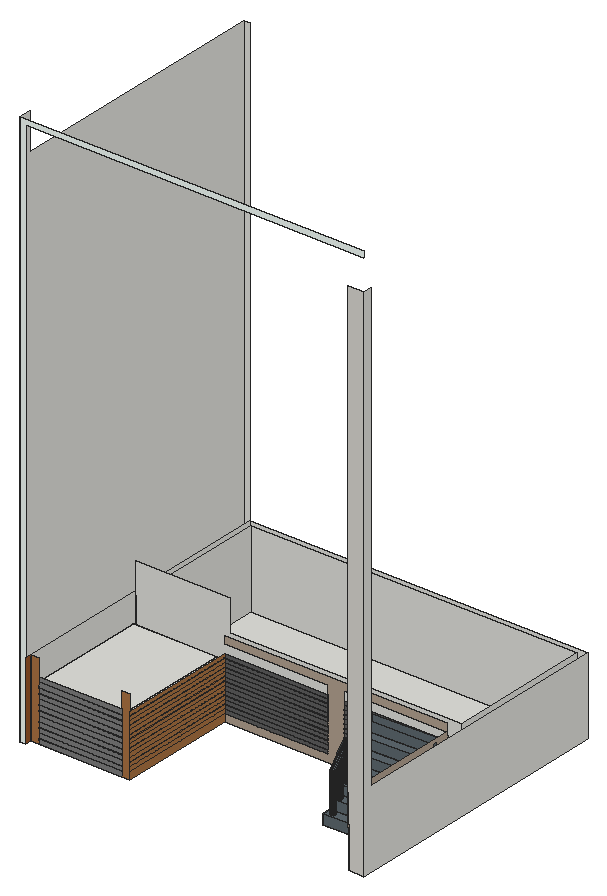
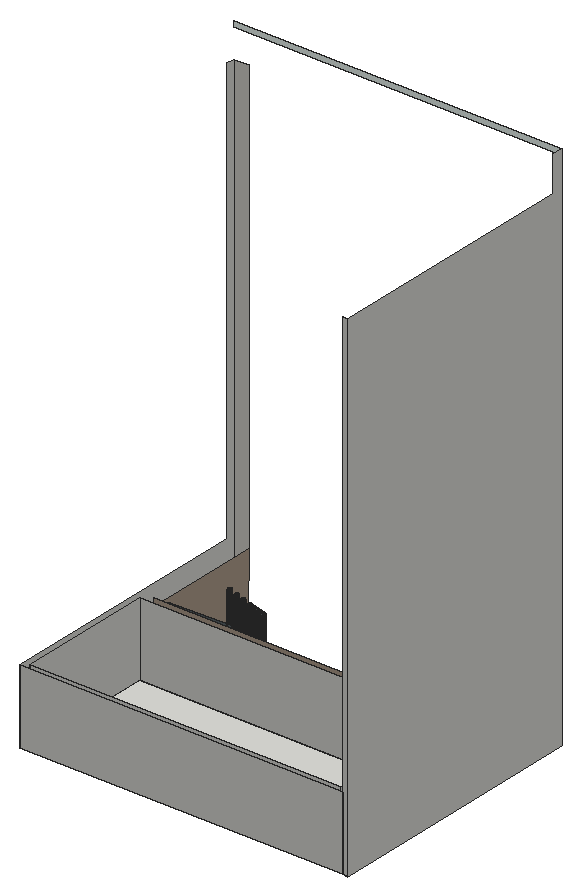
# SketchUp Ruby script. Lengths in inches.
U = 1.inch
M = Sketchup.active_model
def pt(a) = Geom::Point3d.new(a.map { |v| v * U })
def face(e, loops, mat)
  f = e.add_face(loops[0].map { |a| pt(a) })
  loops[1..].each { |l| e.add_face(l.map { |a| pt(a) }).erase! }
  f.material = f.back_material = mat if mat
  f
end
# faces: each face lists its corners as indices into pts; further lists are holes
def faces(e, pts, list, mat = nil) = list.each { |f| face(e, (f[0].is_a?(Array) ? f : [f]).map { |l| l.map { |i| pts[i] } }, mat) }
# xy, xz, yz: faces in a plane at the given z, y or x. An outline is a flat list of corners, or four numbers for a rectangle; further outlines are holes
def ring(l) = l.size == 4 ? [[l[0], l[1]], [l[2], l[1]], [l[2], l[3]], [l[0], l[3]]] : l.each_slice(2).to_a
def flat(e, list, mat, &to3) = list.each { |f| face(e, (f[0].is_a?(Array) ? f : [f]).map { |l| ring(l).map { |u, v| to3.(u, v) } }, mat) }
def xy(e, z, list, mat = nil) = flat(e, list, mat) { |x, y| [x, y, z] }
def xz(e, y, list, mat = nil) = flat(e, list, mat) { |x, z| [x, y, z] }
def yz(e, x, list, mat = nil) = flat(e, list, mat) { |y, z| [x, y, z] }
def lines(e, pts, list) = list.each { |a, b| e.add_line(pt(pts[a]), pt(pts[b])) }
# prism: a flat outline (further loops are holes) pulled along v
def prism(e, loops, v, mat = nil)
  f = face(e, loops, mat); d = Geom::Vector3d.new(v.map { |x| x * U })
  f.pushpull(f.normal.samedirection?(d) ? d.length : -d.length)
end
def box(e, o, s, mat = nil) = prism(e, [[o, [o[0] + s[0], o[1], o[2]], [o[0] + s[0], o[1] + s[1], o[2]], [o[0], o[1] + s[1], o[2]]]], [0, 0, s[2]], mat)
def at(x, y, z, deg = 0) = Geom::Transformation.translation(pt([x, y, z])) * Geom::Transformation.rotation(ORIGIN, Z_AXIS, deg.degrees)
def axes(o, x, y, z) = Geom::Transformation.new([*x, 0, *y, 0, *z, 0, *pt(o).to_a, 1])
def part(name) = M.definitions.add(name)
# library, detail: a bought-in or finely detailed component or shape, given as its bounding box
def library(name, o, s) = part(name).tap { |d| box(d.entities, o, s) }
def detail(e, o, s) = box(e.add_group.entities, o, s)
def put(e, d, t, mat = nil) = e.add_instance(d, t).tap { |i| i.material = mat if mat }
def group(e, t, mat = nil) = e.add_group.tap { |g| g.transformation = t; g.material = mat if mat }.entities
root = M.entities
M.materials.add("[0091_MintCream]").color = [245, 255, 250]
M.materials.add("[0133_Gray]").color = [96, 96, 96]
M.materials.add("[0133_Gray]1").color = [128, 128, 128]
M.materials.add("[0135_DarkGray]").color = [81, 81, 81]
M.materials.add("[Formica Speckled Grey]").color = [94, 105, 111]
M.materials.add("[Terrazzo Tile Light]").color = [219, 217, 210]
M.materials.add("[Travertine Small Tile]").color = [180, 162, 145]
M.materials.add("[Wood Cherry Original]").color = [152, 86, 42]
M.materials.add("[Wood Floor]").color = [172, 116, 67]
xy(root,0,[[0,0,9,432.6875],[[507.6875,0.125,507.6875,191.6875,162.5,191.6875,162.5,9,9,9,9,432.6875,531.4375,432.6875,531.4375,0.125],[18,201.6875,522.4375,423.6875]],[18,201.6875,522.4375,423.6875]])
xy(root,0,[[413.1875,68.82,411.77,84.18,514.98,87.56,516.39,72.2]],"[Formica Speckled Grey]")
xy(root,7.87,[[21,9,150.5,192.6875]])
xy(root,8.37,[[21,9,150.5,192.6875]])
xy(root,14.64,[[[413.1875,68.82,516.39,72.2,514.98,87.56,411.77,84.18],[422.8,73.59,421.86,73.62,420.98,73.8,420.23,74.12,419.65,74.57,419.28,75.11,419.15,75.71,419.26,76.32,419.61,76.9,420.18,77.42,420.92,77.84,421.79,78.125,422.73,78.26,423.67,78.24,424.54,78.05,425.3,77.73,425.875,77.28,426.25,76.74,426.38,76.14,426.26,75.53,425.91,74.95,425.34,74.43,424.6,74.01,423.73,73.73]],[422.8,73.59,421.86,73.62,420.98,73.8,420.23,74.12,419.65,74.57,419.28,75.11,419.15,75.71,419.26,76.32,419.61,76.9,420.18,77.42,420.92,77.84,421.79,78.125,422.73,78.26,423.67,78.24,424.54,78.05,425.3,77.73,425.875,77.28,426.25,76.74,426.38,76.14,426.26,75.53,425.91,74.95,425.34,74.43,424.6,74.01,423.73,73.73],[411.77,84.18,410.35,99.53,513.56,102.92,514.98,87.56]],"[Formica Speckled Grey]")
xy(root,15.24,[[21,9,150.5,192.6875]])
xy(root,15.74,[[21,9,150.5,192.6875]])
xy(root,17.9,[[162.5,191.6875,322.97,192.6875],[347.2,191.6875,507.67,192.6875]])
xy(root,18.4,[[162.5,191.6875,322.97,192.6875],[347.2,191.6875,507.67,192.6875]])
xy(root,23.11,[[21,9,150.5,192.6875]])
xy(root,23.61,[[21,9,150.5,192.6875]])
xy(root,24.3,[[162.5,191.6875,322.97,192.6875],[347.1875,191.6875,507.66,192.6875]])
xy(root,24.8,[[162.5,191.6875,322.97,192.6875],[347.19,191.6875,507.65,192.6875]])
xy(root,29.29,[[[411.77,84.18,514.98,87.56,513.56,102.92,410.35,99.53],[421.38,88.95,420.44,88.97,419.57,89.15,418.8125,89.48,418.23,89.93,417.86,90.47,417.73,91.07,417.84,91.68,418.2,92.26,418.77,92.78,419.51,93.2,420.38,93.48,421.3125,93.62,422.25,93.59,423.125,93.41,423.88,93.09,424.46,92.64,424.83,92.1,424.96,91.5,424.85,90.89,424.49,90.3,423.93,89.79,423.18,89.37,422.3125,89.09]],[421.38,88.95,422.3125,89.09,423.18,89.37,423.93,89.79,424.49,90.3,424.85,90.89,424.96,91.5,424.83,92.1,424.46,92.64,423.88,93.09,423.125,93.41,422.25,93.59,421.3125,93.62,420.38,93.48,419.51,93.2,418.77,92.78,418.2,92.26,417.84,91.68,417.73,91.07,417.86,90.47,418.23,89.93,418.8125,89.48,419.57,89.15,420.44,88.97],[410.35,99.53,408.9375,114.89,512.14,118.28,513.56,102.92]],"[Formica Speckled Grey]")
xy(root,30.7,[[162.5,191.6875,322.97,192.6875],[347.17,191.6875,507.64,192.6875]])
xy(root,30.98,[[21,9,150.5,192.6875]])
xy(root,31.2,[[162.5,191.6875,322.97,192.6875],[347.17,191.6875,507.64,192.6875]])
xy(root,31.48,[[21,9,150.5,192.6875]])
xy(root,37.1,[[162.5,191.6875,322.97,192.6875],[347.15,191.6875,507.62,192.6875]])
xy(root,37.6,[[162.5,191.6875,322.97,192.6875],[347.15,191.6875,507.62,192.6875]])
xy(root,38.85,[[21,9,150.5,192.6875]])
xy(root,39.35,[[21,9,150.5,192.6875]])
xy(root,43.5,[[162.5,191.6875,322.97,192.6875],[347.14,191.6875,507.61,192.6875]])
xy(root,43.93,[[[410.35,99.53,513.56,102.92,512.14,118.28,408.9375,114.89],[419.96,104.31,419.03,104.33,418.15,104.51,417.4,104.84,416.82,105.29,416.45,105.83,416.3125,106.43,416.43,107.04,416.78,107.62,417.35,108.14,418.09,108.56,418.96,108.84,419.9,108.98,420.83,108.95,421.71,108.77,422.46,108.45,423.04,108,423.41,107.46,423.55,106.86,423.43,106.25,423.08,105.66,422.51,105.15,421.77,104.73,420.9,104.44]],[419.96,104.31,420.9,104.44,421.77,104.73,422.51,105.15,423.08,105.66,423.43,106.25,423.55,106.86,423.41,107.46,423.04,108,422.46,108.45,421.71,108.77,420.83,108.95,419.9,108.98,418.96,108.84,418.09,108.56,417.35,108.14,416.78,107.62,416.43,107.04,416.3125,106.43,416.45,105.83,416.82,105.29,417.4,104.84,418.15,104.51,419.03,104.33],[408.9375,114.89,407.52,130.25,510.73,133.63,512.14,118.28]],"[Formica Speckled Grey]")
xy(root,44,[[162.5,191.6875,322.97,192.6875],[347.14,191.6875,507.6,192.6875]])
xy(root,46.73,[[21,9,150.5,192.6875]])
xy(root,47.23,[[21,9,150.5,192.6875]])
xy(root,49.9,[[162.5,191.6875,322.97,192.6875],[347.12,191.6875,507.59,192.6875]])
xy(root,50.4,[[162.5,191.6875,322.97,192.6875],[347.12,191.6875,507.59,192.6875]])
xy(root,54.6,[[21,9,150.5,192.6875]])
xy(root,55.1,[[21,9,150.5,192.6875]])
xy(root,56.3,[[162.5,191.6875,322.97,192.6875],[347.1,191.6875,507.57,192.6875]])
xy(root,56.8,[[347.1,191.6875,507.57,192.6875],[162.5,192.0625,322.97,192.6875]])
xy(root,58.57,[[[408.9375,114.89,512.14,118.28,510.73,133.63,407.52,130.25],[418.55,119.67,417.61,119.69,416.74,119.87,415.98,120.2,415.4,120.65,415.03,121.1875,414.9,121.78,415.01,122.4,415.37,122.98,415.93,123.5,416.68,123.91,417.55,124.2,418.48,124.34,419.42,124.3125,420.29,124.13,421.05,123.8,421.63,123.36,422,122.81,422.13,122.22,422.02,121.61,421.66,121.02,421.09,120.5,420.35,120.09,419.48,119.8]],[418.55,119.67,419.48,119.8,420.35,120.09,421.09,120.5,421.66,121.02,422.02,121.61,422.13,122.22,422,122.81,421.63,123.36,421.05,123.8,420.29,124.13,419.42,124.3125,418.48,124.34,417.55,124.2,416.68,123.91,415.93,123.5,415.37,122.98,415.01,122.4,414.9,121.78,415.03,121.1875,415.4,120.65,415.98,120.2,416.74,119.87,417.61,119.69],[407.52,130.25,406.11,145.61,509.3125,148.99,510.73,133.63]],"[Formica Speckled Grey]")
xy(root,62.47,[[21,9,150.5,192.6875]])
xy(root,62.7,[[347.09,191.6875,507.56,192.6875],[162.5,192.0625,322.97,192.6875]])
xy(root,62.97,[[21,9,150.5,192.6875]])
xy(root,63.2,[[347.09,191.6875,507.55,192.6875],[162.5,192.0625,322.97,192.6875]])
xy(root,69.1,[[347.07,191.6875,507.54,192.6875],[162.5,192.0625,322.97,192.6875]])
xy(root,69.6,[[347.07,191.6875,507.54,192.6875],[162.5,192.0625,322.97,192.6875]])
xy(root,70.34,[[21,9,150.5,192.6875]])
xy(root,70.84,[[21,9,150.5,192.6875]])
xy(root,73.21,[[[407.52,130.25,510.73,133.63,509.3125,148.99,406.11,145.61],[417.13,135.03,416.19,135.05,415.32,135.23,414.56,135.56,413.98,136.01,413.61,136.55,413.48,137.14,413.6,137.75,413.95,138.34,414.52,138.86,415.26,139.27,416.13,139.56,417.0625,139.69,418,139.67,418.875,139.49,419.63,139.16,420.21,138.71,420.58,138.17,420.71,137.58,420.6,136.97,420.25,136.38,419.68,135.86,418.93,135.45,418.07,135.16]],[417.13,135.03,418.07,135.16,418.93,135.45,419.68,135.86,420.25,136.38,420.6,136.97,420.71,137.58,420.58,138.17,420.21,138.71,419.63,139.16,418.875,139.49,418,139.67,417.0625,139.69,416.13,139.56,415.26,139.27,414.52,138.86,413.95,138.34,413.6,137.75,413.48,137.14,413.61,136.55,413.98,136.01,414.56,135.56,415.32,135.23,416.19,135.05],[406.11,145.61,404.69,160.97,507.9,164.35,509.3125,148.99]],"[Formica Speckled Grey]")
xy(root,75.5,[[347.05,191.6875,507.52,192.6875],[162.5,192.0625,322.97,192.6875]])
xy(root,76,[[347.05,191.6875,507.52,192.6875],[162.5,192.0625,322.97,192.6875]])
xy(root,78.21,[[21,9,150.5,192.6875]])
xy(root,78.71,[[21,9,150.5,192.6875]])
xy(root,81.9,[[347.04,191.6875,507.51,192.6875],[162.5,192.0625,322.97,192.6875]])
xy(root,82.4,[[347.04,191.6875,507.5,192.6875],[162.5,192.0625,322.97,192.6875]])
xy(root,86.08,[[21,9,150.5,192.6875]])
xy(root,86.58,[[21,9,150.5,192.6875]])
xy(root,87.86,[[[406.11,145.61,509.3125,148.99,507.9,164.35,404.69,160.97],[415.72,150.39,414.78,150.41,413.9,150.59,413.15,150.92,412.57,151.36,412.2,151.91,412.07,152.5,412.18,153.11,412.53,153.7,413.1,154.22,413.85,154.63,414.71,154.92,415.65,155.05,416.59,155.03,417.46,154.85,418.22,154.52,418.8,154.07,419.17,153.53,419.3,152.9375,419.18,152.32,418.83,151.74,418.26,151.22,417.52,150.81,416.65,150.52]],[415.72,150.39,416.65,150.52,417.52,150.81,418.26,151.22,418.83,151.74,419.18,152.32,419.3,152.9375,419.17,153.53,418.8,154.07,418.22,154.52,417.46,154.85,416.59,155.03,415.65,155.05,414.71,154.92,413.85,154.63,413.1,154.22,412.53,153.7,412.18,153.11,412.07,152.5,412.2,151.91,412.57,151.36,413.15,150.92,413.9,150.59,414.78,150.41],[404.69,160.97,403.27,176.33,506.48,179.71,507.9,164.35]],"[Formica Speckled Grey]")
xy(root,88.3,[[347.02,191.6875,507.49,192.6875],[162.5,192.0625,322.97,192.6875]])
xy(root,88.8,[[347.02,191.6875,507.49,192.6875],[162.5,192.0625,322.97,192.6875]])
xz(root,0,[[0,0,9,0,9,858,531.4375,858,531.4375,866.75,0,866.75]],"[0091_MintCream]")
xz(root,0.125,[[507.6875,0,531.4375,0,531.4375,810,507.4375,810,507.4375,108,507.6875,12]],"[Terrazzo Tile Light]")
xz(root,9,[[21,0,150.5,7.87],[21,8.37,150.5,15.24],[21,15.74,150.5,23.11],[21,23.61,150.5,30.98],[21,31.48,150.5,38.85],
  [21,39.35,150.5,46.73],[21,47.23,150.5,54.6],[21,55.1,150.5,62.47],[21,62.97,150.5,70.34],[21,70.84,150.5,78.21],
  [21,78.71,150.5,86.08],[21,86.58,150.5,93.95]],"[0133_Gray]1")
xz(root,9,[[9,0,21,120],[150.5,0,162.5,120]],"[Wood Floor]")
xz(root,191.6875,[[162.5,12,322.97,17.9],[347.22,12,507.6875,12,507.67,17.9,347.2,17.9],[162.5,18.4,322.97,24.3],[347.2,18.4,507.67,18.4,507.66,24.3,347.1875,24.3],[162.5,24.8,322.97,30.7],
  [347.19,24.8,507.65,24.8,507.64,30.7,347.17,30.7],[162.5,31.2,322.97,37.1],[347.17,31.2,507.64,31.2,507.62,37.1,347.15,37.1],[162.5,37.6,322.97,43.5],[347.15,37.6,507.62,37.6,507.61,43.5,347.14,43.5],
  [162.5,44,322.97,49.9],[347.14,44,507.6,44,507.59,49.9,347.12,49.9],[162.5,50.4,322.97,56.3],[347.12,50.4,507.59,50.4,507.57,56.3,347.1,56.3],[347.1,56.8,507.57,56.8,507.56,62.7,347.09,62.7],
  [347.09,63.2,507.55,63.2,507.54,69.1,347.07,69.1],[347.07,69.6,507.54,69.6,507.52,75.5,347.05,75.5],[347.05,76,507.52,76,507.51,81.9,347.04,81.9],[347.04,82.4,507.5,82.4,507.49,88.3,347.02,88.3],[347.02,88.8,507.49,88.8,507.47,94.7,347,94.7]],"[0133_Gray]")
xz(root,191.6875,[[162.5,0,507.6875,0,507.6875,12,347.22,12,347.2,17.9,347.2,18.4,347.1875,24.3,347.19,24.8,347.17,30.7,347.17,31.2,347.15,37.1,347.15,37.6,347.14,43.5,347.14,44,347.12,49.9,347.12,50.4,347.1,56.3,347.1,56.8,347.09,62.7,347.09,63.2,347.07,69.1,347.07,69.6,347.05,75.5,347.05,76,347.04,81.9,347.04,82.4,347.02,88.3,347.02,88.8,347,94.7,347,95.2,346.99,101.1,346.99,101.6,346.97,108,507.4375,108,507.4375,120,162.5,120,162.5,108,322.97,108,322.97,12,162.5,12]],"[Travertine Small Tile]")
xz(root,192.0625,[[162.5,56.8,322.97,62.7],[162.5,63.2,322.97,69.1],[162.5,69.6,322.97,75.5],[162.5,76,322.97,81.9],[162.5,82.4,322.97,88.3],
  [162.5,88.8,322.97,94.7]],"[0133_Gray]")
xz(root,192.6875,[[347.2,17.9,507.67,18.4],[347.1875,24.3,507.66,24.3,507.65,24.8,347.19,24.8],[347.17,30.7,507.64,31.2],[347.15,37.1,507.62,37.6],[347.14,43.5,507.61,43.5,507.6,44,347.14,44],
  [347.12,49.9,507.59,50.4],[347.1,56.3,507.57,56.8],[347.09,62.7,507.56,62.7,507.55,63.2,347.09,63.2],[347.07,69.1,507.54,69.6],[347.05,75.5,507.52,76],
  [347.04,81.9,507.51,81.9,507.5,82.4,347.04,82.4],[347.02,88.3,507.49,88.8]])
xz(root,192.6875,[[21,7.87,150.5,8.37],[21,15.24,150.5,15.74],[162.5,17.9,322.97,18.4],[21,23.11,150.5,23.61],[162.5,24.3,322.97,24.8],
  [162.5,30.7,322.97,31.2],[21,30.98,150.5,31.48],[162.5,37.1,322.97,37.6],[21,38.85,150.5,39.35],[162.5,43.5,322.97,44],
  [21,46.73,150.5,47.23],[162.5,49.9,322.97,50.4],[21,54.6,150.5,55.1],[162.5,56.3,322.97,56.8],[21,62.47,150.5,62.97],
  [162.5,62.7,322.97,63.2],[162.5,69.1,322.97,69.6],[21,70.34,150.5,70.84],[162.5,75.5,322.97,76],[21,78.21,150.5,78.71],
  [162.5,81.9,322.97,82.4],[21,86.08,150.5,86.58],[162.5,88.3,322.97,88.8]],"[0135_DarkGray]")
xz(root,201.6875,[[18,0,18,168,162.5,168,162.5,120,522.4375,120,522.4375,0]])
xz(root,423.6875,[[18,0,522.4375,120]])
xz(root,432.6875,[[0,0,9,810],[9,0,531.4375,120]])
yz(root,0,[[0,0,0,866.75,18,866.75,18,810,432.6875,810,432.6875,0]])
yz(root,9,[[9,0,432.6875,120]])
yz(root,9,[[0,0,9,120]],"[Wood Cherry Original]")
yz(root,18,[[201.6875,0,423.6875,120]])
yz(root,21,[[9,7.87,192.6875,8.37],[9,15.24,192.6875,15.74],[9,23.11,192.6875,23.61],[9,30.98,192.6875,31.48],[9,38.85,192.6875,39.35],
  [9,46.73,192.6875,47.23],[9,54.6,192.6875,55.1],[9,62.47,192.6875,62.97],[9,70.34,192.6875,70.84],[9,78.21,192.6875,78.71],
  [9,86.08,192.6875,86.58]])
yz(root,150.5,[[9,7.87,192.6875,8.37],[9,15.24,192.6875,15.74],[9,23.11,192.6875,23.61],[9,30.98,192.6875,31.48],[9,38.85,192.6875,39.35],
  [9,46.73,192.6875,47.23],[9,54.6,192.6875,55.1],[9,62.47,192.6875,62.97],[9,70.34,192.6875,70.84],[9,78.21,192.6875,78.71],
  [9,86.08,192.6875,86.58]],"[Wood Floor]")
yz(root,162.5,[[9,0,191.6875,12],[9,12,191.6875,17.9],[9,17.9,192.6875,18.4],[9,18.4,191.6875,24.3],[9,24.3,192.6875,24.8],
  [9,24.8,191.6875,30.7],[9,30.7,192.6875,31.2],[9,31.2,191.6875,37.1],[9,37.1,192.6875,37.6],[9,37.6,191.6875,43.5],
  [9,43.5,192.6875,44],[9,44,191.6875,49.9],[9,49.9,192.6875,50.4],[9,50.4,191.6875,56.3],[9,56.3,192.6875,56.8],
  [9,56.8,192.0625,62.7],[9,62.7,192.6875,63.2],[9,63.2,192.0625,69.1],[9,69.1,192.6875,69.6],[9,69.6,192.0625,75.5],
  [9,75.5,192.6875,76],[9,76,192.0625,81.9],[9,81.9,192.6875,82.4],[9,82.4,192.0625,88.3],[9,88.3,192.6875,88.8],
  [9,88.8,192.0625,94.7]],"[Wood Floor]")
yz(root,322.97,[[191.6875,17.9,192.6875,18.4],[191.6875,24.3,192.6875,24.8],[191.6875,30.7,192.6875,31.2],[191.6875,37.1,192.6875,37.6],[191.6875,43.5,192.6875,44],
  [191.6875,49.9,192.6875,50.4],[191.6875,56.3,192.6875,56.8],[191.6875,56.8,192.0625,62.7],[191.6875,62.7,192.6875,63.2],[191.6875,63.2,192.0625,69.1],
  [191.6875,69.1,192.6875,69.6],[191.6875,69.6,192.0625,75.5],[191.6875,75.5,192.6875,76],[191.6875,76,192.0625,81.9],[191.6875,81.9,192.6875,82.4],
  [191.6875,82.4,192.0625,88.3],[191.6875,88.3,192.6875,88.8],[191.6875,88.8,192.0625,94.7]])
yz(root,347.02,[[191.6875,88.3,192.6875,88.8]])
yz(root,347.04,[[191.6875,81.9,192.6875,82.4]])
yz(root,347.05,[[191.6875,75.5,192.6875,76]])
yz(root,347.07,[[191.6875,69.1,192.6875,69.6]])
yz(root,347.09,[[191.6875,62.7,192.6875,63.2]])
yz(root,347.1,[[191.6875,56.3,192.6875,56.8]])
yz(root,347.12,[[191.6875,49.9,192.6875,50.4]])
yz(root,347.14,[[191.6875,43.5,192.6875,44]])
yz(root,347.15,[[191.6875,37.1,192.6875,37.6]])
yz(root,347.17,[[191.6875,30.7,192.6875,31.2]])
yz(root,347.2,[[191.6875,17.9,192.6875,18.4]])
yz(root,507.6875,[[0.125,0,191.6875,12]],"[Travertine Small Tile]")
yz(root,522.4375,[[201.6875,0,423.6875,120]])
yz(root,531.4375,[[0.125,0,432.6875,0,432.6875,120,13,120,13,810,0.125,810]])
p = [[411.77,84.18,0],[413.1875,68.82,0],[413.1875,68.82,14.64],[411.77,84.18,14.64],[516.39,72.2,0],[516.39,72.2,14.64],
  [514.98,87.56,0],[514.98,87.56,14.64],[507.64,192.6875,30.7],[507.64,191.6875,30.7],[507.65,191.6875,24.8],[507.65,192.6875,24.8],
  [507.66,192.6875,24.3],[507.66,191.6875,24.3],[507.67,191.6875,18.4],[507.67,192.6875,18.4],[507.67,192.6875,17.9],[507.67,191.6875,17.9],
  [507.6875,191.6875,12],[507.6875,0.125,12],[507.4375,0.125,108],[507.4375,191.6875,108],[507.45,191.6875,101.6],[507.45,192.6875,101.6],
  [507.46,192.6875,101.1],[507.46,191.6875,101.1],[507.47,191.6875,95.2],[507.47,192.6875,95.2],[507.47,192.6875,94.7],[507.47,191.6875,94.7],
  [507.49,191.6875,88.8],[507.49,192.6875,88.8],[507.49,192.6875,88.3],[507.49,191.6875,88.3],[507.5,191.6875,82.4],[507.5,192.6875,82.4],
  [507.51,192.6875,81.9],[507.51,191.6875,81.9],[507.52,191.6875,76],[507.52,192.6875,76],[507.52,192.6875,75.5],[507.52,191.6875,75.5],
  [507.54,191.6875,69.6],[507.54,192.6875,69.6],[507.54,192.6875,69.1],[507.54,191.6875,69.1],[507.55,191.6875,63.2],[507.55,192.6875,63.2],
  [507.56,192.6875,62.7],[507.56,191.6875,62.7],[507.57,191.6875,56.8],[507.57,192.6875,56.8],[507.57,192.6875,56.3],[507.57,191.6875,56.3],
  [507.59,191.6875,50.4],[507.59,192.6875,50.4],[507.59,192.6875,49.9],[507.59,191.6875,49.9],[507.6,191.6875,44],[507.6,192.6875,44],
  [507.61,192.6875,43.5],[507.61,191.6875,43.5],[507.62,191.6875,37.6],[507.62,192.6875,37.6],[507.62,192.6875,37.1],[507.62,191.6875,37.1],
  [507.64,191.6875,31.2],[507.64,192.6875,31.2],[420.98,73.8,14.64],[421.86,73.62,14.64],[421.86,73.62,75.8125],[420.98,73.8,75.51],
  [422.8,73.59,14.64],[422.8,73.59,75.94],[423.73,73.73,14.64],[423.73,73.73,75.89],[424.6,74.01,14.64],[424.6,74.01,75.65],
  [420.23,74.12,14.64],[420.23,74.12,75.05],[425.34,74.43,14.64],[425.34,74.43,75.24],[419.65,74.57,14.64],[419.65,74.57,74.46],
  [425.91,74.95,14.64],[425.91,74.95,74.7],[419.28,75.11,14.64],[419.28,75.11,73.79],[426.26,75.53,14.64],[426.26,75.53,74.05],
  [419.15,75.71,14.64],[419.15,75.71,73.08],[426.38,76.14,14.64],[426.38,76.14,73.35],[419.26,76.32,14.64],[419.26,76.32,72.375],
  [426.25,76.74,14.64],[426.25,76.74,72.64],[419.61,76.9,14.64],[419.61,76.9,71.73],[425.875,77.28,14.64],[425.875,77.28,71.97],
  [420.18,77.42,14.64],[420.18,77.42,71.19],[425.3,77.73,14.64],[425.3,77.73,71.38],[420.92,77.84,14.64],[420.92,77.84,70.78],
  [424.54,78.05,14.64],[424.54,78.05,70.92],[421.79,78.125,14.64],[421.79,78.125,70.54],[422.73,78.26,14.64],[422.73,78.26,70.48],
  [423.67,78.24,14.64],[423.67,78.24,70.61],[410.35,99.53,14.64],[411.77,84.18,29.29],[410.35,99.53,29.29],[514.98,87.56,29.29],
  [513.56,102.92,14.64],[513.56,102.92,29.29],[347.1875,192.6875,24.3],[347.19,192.6875,24.8],[347.19,191.6875,24.8],[347.1875,191.6875,24.3],
  [419.57,89.15,29.29],[420.44,88.97,29.29],[420.44,88.97,90.46],[419.57,89.15,90.15],[421.38,88.95,29.29],[421.38,88.95,90.59],
  [422.3125,89.09,29.29],[422.3125,89.09,90.53],[423.18,89.37,29.29],[423.18,89.37,90.29],[418.8125,89.48,29.29],[418.8125,89.48,89.6875],
  [423.93,89.79,29.29],[423.93,89.79,89.88],[418.23,89.93,29.29],[418.23,89.93,89.1],[424.49,90.3,29.29],[424.49,90.3,89.34],
  [417.86,90.47,29.29],[417.86,90.47,88.43],[424.85,90.89,29.29],[424.85,90.89,88.69],[417.73,91.07,29.29],[417.73,91.07,87.72],
  [424.96,91.5,29.29],[424.96,91.5,87.99],[417.84,91.68,29.29],[417.84,91.68,87.02],[424.83,92.1,29.29],[424.83,92.1,87.28],
  [418.2,92.26,29.29],[418.2,92.26,86.37],[424.46,92.64,29.29],[424.46,92.64,86.61],[418.77,92.78,29.29],[418.77,92.78,85.83],
  [423.88,93.09,29.29],[423.88,93.09,86.02],[419.51,93.2,29.29],[419.51,93.2,85.42],[423.125,93.41,29.29],[423.125,93.41,85.56],
  [420.38,93.48,29.29],[420.38,93.48,85.18],[422.25,93.59,29.29],[422.25,93.59,85.25],[421.3125,93.62,29.29],[421.3125,93.62,85.125],
  [408.9375,114.89,29.29],[410.35,99.53,43.93],[408.9375,114.89,43.93],[513.56,102.92,43.93],[512.14,118.28,29.29],[512.14,118.28,43.93],
  [418.15,104.51,43.93],[419.03,104.33,43.93],[419.03,104.33,105.1],[418.15,104.51,104.79],[419.96,104.31,43.93],[419.96,104.31,105.23],
  [420.9,104.44,43.93],[420.9,104.44,105.17],[421.77,104.73,43.93],[421.77,104.73,104.93],[417.4,104.84,43.93],[417.4,104.84,104.33],
  [422.51,105.15,43.93],[422.51,105.15,104.52],[416.82,105.29,43.93],[416.82,105.29,103.74],[423.08,105.66,43.93],[423.08,105.66,103.98],
  [416.45,105.83,43.93],[416.45,105.83,103.07],[423.43,106.25,43.93],[423.43,106.25,103.34],[416.3125,106.43,43.93],[416.3125,106.43,102.36],
  [423.55,106.86,43.93],[423.55,106.86,102.63],[416.43,107.04,43.93],[416.43,107.04,101.66],[423.41,107.46,43.93],[423.41,107.46,101.92],
  [416.78,107.62,43.93],[416.78,107.62,101.01],[423.04,108,43.93],[423.04,108,101.25],[417.35,108.14,43.93],[417.35,108.14,100.47],
  [422.46,108.45,43.93],[422.46,108.45,100.66],[418.09,108.56,43.93],[418.09,108.56,100.06],[421.71,108.77,43.93],[421.71,108.77,100.2],
  [418.96,108.84,43.93],[418.96,108.84,99.82],[419.9,108.98,43.93],[419.9,108.98,99.77],[420.83,108.95,43.93],[420.83,108.95,99.9],
  [407.52,130.25,43.93],[408.9375,114.89,58.57],[407.52,130.25,58.57],[512.14,118.28,58.57],[510.73,133.63,43.93],[510.73,133.63,58.57],
  [416.74,119.87,58.57],[417.61,119.69,58.57],[417.61,119.69,119.74],[416.74,119.87,119.4375],[418.55,119.67,58.57],[418.55,119.67,119.87],
  [419.48,119.8,58.57],[419.48,119.8,119.8125],[420.35,120.09,58.57],[420.35,120.09,119.57],[415.98,120.2,58.57],[415.98,120.2,118.97],
  [421.09,120.5,58.57],[421.09,120.5,119.17],[415.4,120.65,58.57],[415.4,120.65,118.39],[421.66,121.02,58.57],[421.66,121.02,118.625],
  [415.03,121.1875,58.57],[415.03,121.1875,117.71],[422.02,121.61,58.57],[422.02,121.61,117.98],[414.9,121.78,58.57],[414.9,121.78,117],
  [422.13,122.22,58.57],[422.13,122.22,117.28],[415.01,122.4,58.57],[415.01,122.4,116.3],[422,122.81,58.57],[422,122.81,116.57],
  [415.37,122.98,58.57],[415.37,122.98,115.66],[421.63,123.36,58.57],[421.63,123.36,115.89],[415.93,123.5,58.57],[415.93,123.5,115.11],
  [421.05,123.8,58.57],[421.05,123.8,115.31],[416.68,123.91,58.57],[416.68,123.91,114.71],[420.29,124.13,58.57],[420.29,124.13,114.84],
  [417.55,124.2,58.57],[417.55,124.2,114.47],[419.42,124.3125,58.57],[419.42,124.3125,114.54],[418.48,124.34,58.57],[418.48,124.34,114.41],
  [406.11,145.61,58.57],[407.52,130.25,73.21],[406.11,145.61,73.21],[510.73,133.63,73.21],[509.3125,148.99,58.57],[509.3125,148.99,73.21],
  [420.49,92.23,83.99],[419.61,92.06,84.33],[421.43,92.34,83.9],[422.36,92.375,84.09],[423.22,92.34,84.53],[418.85,91.83,84.92],
  [423.96,92.23,85.2],[418.26,91.57,85.71],[424.51,92.05,86.05],[417.88,91.29,86.64],[424.85,91.83,87.02],[417.74,91,87.66],
  [416.19,135.05,73.21],[417.13,135.03,73.21],[417.13,135.03,134.51],[416.19,135.05,134.38],[418.07,135.16,73.21],[418.07,135.16,134.46],
  [415.32,135.23,73.21],[415.32,135.23,134.08],[414.56,135.56,73.21],[414.56,135.56,133.62],[418.93,135.45,73.21],[418.93,135.45,134.22],
  [419.68,135.86,73.21],[419.68,135.86,133.81],[413.98,136.01,73.21],[413.98,136.01,133.03],[420.25,136.38,73.21],[420.25,136.38,133.27],
  [413.61,136.55,73.21],[413.61,136.55,132.36],[420.6,136.97,73.21],[420.6,136.97,132.62],[413.48,137.14,73.21],[413.48,137.14,131.65],
  [420.71,137.58,73.21],[420.71,137.58,131.92],[413.6,137.75,73.21],[413.6,137.75,130.94],[420.58,138.17,73.21],[420.58,138.17,131.21],
  [413.95,138.34,73.21],[413.95,138.34,130.3],[420.21,138.71,73.21],[420.21,138.71,130.54],[414.52,138.86,73.21],[414.52,138.86,129.76],
  [419.63,139.16,73.21],[419.63,139.16,129.95],[415.26,139.27,73.21],[415.26,139.27,129.35],[418.875,139.49,73.21],[418.875,139.49,129.49],
  [416.13,139.56,73.21],[416.13,139.56,129.11],[418,139.67,73.21],[418,139.67,129.18],[417.0625,139.69,73.21],[417.0625,139.69,129.05],
  [404.69,160.97,73.21],[406.11,145.61,87.86],[404.69,160.97,87.86],[509.3125,148.99,87.86],[507.9,164.35,73.21],[507.9,164.35,87.86],
  [420.01,107.7,98.55],[419.08,107.59,98.63],[420.95,107.73,98.73],[418.2,107.41,98.98],[421.81,107.69,99.17],[417.4375,107.1875,99.5625],
  [422.54,107.59,99.84],[416.85,106.93,100.35],[423.1,107.41,100.69],[416.46,106.64,101.28],[423.4375,107.1875,101.67],[416.32,106.36,102.3],
  [424.96,91.56,88.05],[417.84,90.74,88.6875],[413.9,150.59,87.86],[414.78,150.41,87.86],[414.78,150.41,149.03],[413.9,150.59,148.72],
  [415.72,150.39,87.86],[415.72,150.39,149.16],[416.65,150.52,87.86],[416.65,150.52,149.1],[417.52,150.81,87.86],[417.52,150.81,148.86],
  [413.15,150.92,87.86],[413.15,150.92,148.26],[418.26,151.22,87.86],[418.26,151.22,148.45],[412.57,151.36,87.86],[412.57,151.36,147.67],
  [418.83,151.74,87.86],[418.83,151.74,147.91],[412.2,151.91,87.86],[412.2,151.91,147],[419.18,152.32,87.86],[419.18,152.32,147.26],
  [412.07,152.5,87.86],[412.07,152.5,146.29],[419.3,152.9375,87.86],[419.3,152.9375,146.5625],[412.18,153.11,87.86],[412.18,153.11,145.59],
  [419.17,153.53,87.86],[419.17,153.53,145.85],[412.53,153.7,87.86],[412.53,153.7,144.94],[418.8,154.07,87.86],[418.8,154.07,145.18],
  [413.1,154.22,87.86],[413.1,154.22,144.4],[418.22,154.52,87.86],[418.22,154.52,144.59],[413.85,154.63,87.86],[413.85,154.63,143.99],
  [417.46,154.85,87.86],[417.46,154.85,144.13],[414.71,154.92,87.86],[414.71,154.92,143.75],[416.59,155.03,87.86],[416.59,155.03,143.82],
  [415.65,155.05,87.86],[415.65,155.05,143.69],[403.27,176.33,87.86],[404.69,160.97,102.5],[403.27,176.33,102.5],[507.9,164.35,102.5],
  [506.48,179.71,87.86],[506.48,179.71,102.5],[424.8125,91.28,89.07],[418.18,90.51,89.66],[424.43,91,90],[418.73,90.34,90.51],
  [423.84,90.74,90.79],[419.47,90.23,91.18],[423.08,90.51,91.375],[420.33,90.19,91.62],[422.2,90.34,91.72],[421.26,90.23,91.81]]
faces(root,p,[[0,1,2,3],[1,4,5,2],[4,6,7,5],[6,0,3,7],[68,69,70,71],[69,72,73,70],[72,74,75,73],[74,76,77,75],
  [78,68,71,79],[76,80,81,77],[82,78,79,83],[80,84,85,81],[86,82,83,87],[84,88,89,85],[90,86,87,91],[88,92,93,89],
  [94,90,91,95],[92,96,97,93],[98,94,95,99],[96,100,101,97],[102,98,99,103],[100,104,105,101],[106,102,103,107],[104,108,109,105],
  [110,106,107,111],[112,110,111,113],[108,114,115,109],[114,112,113,115],[116,3,117,118],[3,7,119,117],[7,120,121,119],[120,116,118,121],
  [126,127,128,129],[127,130,131,128],[130,132,133,131],[132,134,135,133],[136,126,129,137],[134,138,139,135],[140,136,137,141],[138,142,143,139],
  [144,140,141,145],[142,146,147,143],[148,144,145,149],[146,150,151,147],[152,148,149,153],[150,154,155,151],[156,152,153,157],[154,158,159,155],
  [160,156,157,161],[158,162,163,159],[164,160,161,165],[162,166,167,163],[168,164,165,169],[166,170,171,167],[172,168,169,173],[170,172,173,171],
  [174,118,175,176],[118,121,177,175],[121,178,179,177],[178,174,176,179],[180,181,182,183],[181,184,185,182],[184,186,187,185],[186,188,189,187],
  [190,180,183,191],[188,192,193,189],[194,190,191,195],[192,196,197,193],[198,194,195,199],[196,200,201,197],[202,198,199,203],[200,204,205,201],
  [206,202,203,207],[204,208,209,205],[210,206,207,211],[208,212,213,209],[214,210,211,215],[212,216,217,213],[218,214,215,219],[216,220,221,217],
  [222,218,219,223],[224,222,223,225],[220,226,227,221],[226,224,225,227],[228,176,229,230],[176,179,231,229],[179,232,233,231],[232,228,230,233],
  [234,235,236,237],[235,238,239,236],[238,240,241,239],[240,242,243,241],[244,234,237,245],[242,246,247,243],[248,244,245,249],[246,250,251,247],
  [252,248,249,253],[250,254,255,251],[256,252,253,257],[254,258,259,255],[260,256,257,261],[258,262,263,259],[264,260,261,265],[262,266,267,263],
  [268,264,265,269],[266,270,271,267],[272,268,269,273],[270,274,275,271],[276,272,273,277],[274,278,279,275],[280,276,277,281],[278,280,281,279],
  [282,230,283,284],[230,233,285,283],[233,286,287,285],[286,282,284,287],[165,169,288,111,107,289],[169,173,290,113,111,288],[173,171,291,115,113,290],[171,167,292,109,115,291],
  [161,165,289,107,103,293],[167,163,294,105,109,292],[295,157,161,293,103,99],[105,294,163,159,296,101],[297,153,157,295,99,95],[101,296,159,155,298,97],[299,149,153,297,95,91],[97,298,155,151,93],
  [87,145,149,299,91],[300,301,302,303],[301,304,305,302],[306,300,303,307],[308,306,307,309],[304,310,311,305],[310,312,313,311],[314,308,309,315],
  [312,316,317,313],[318,314,315,319],[316,320,321,317],[322,318,319,323],[320,324,325,321],[326,322,323,327],[324,328,329,325],[330,326,327,331],
  [328,332,333,329],[334,330,331,335],[332,336,337,333],[338,334,335,339],[336,340,341,337],[342,338,339,343],[340,344,345,341],[346,342,343,347],
  [344,346,347,345],[348,284,349,350],[284,287,351,349],[287,352,353,351],[352,348,350,353],[89,93,151,147],[83,141,145,87],[85,89,147,143],
  [79,137,141,83],[81,85,143,139],[79,71,129,137],[77,81,139,135],[71,70,128,129],[75,77,135,133],[70,73,131,128],[73,75,133,131],
  [223,225,354,173,169,355],[225,227,356,171,173,354],[219,223,355,169,165,357],[227,221,358,167,171,356],[215,219,357,165,161,359],[221,217,360,163,167,358],[361,211,215,359,161,157],[163,360,217,213,362,159],
  [363,207,211,361,157,153],[159,362,213,209,364,155],[365,203,207,363,153,149],[155,364,209,205,366,151],[367,199,203,365,149,145],[368,369,370,371],[369,372,373,370],[372,374,375,373],
  [374,376,377,375],[378,368,371,379],[376,380,381,377],[382,378,379,383],[380,384,385,381],[386,382,383,387],[384,388,389,385],[390,386,387,391],
  [388,392,393,389],[394,390,391,395],[392,396,397,393],[398,394,395,399],[396,400,401,397],[402,398,399,403],[400,404,405,401],[406,402,403,407],
  [404,408,409,405],[410,406,407,411],[408,412,413,409],[414,410,411,415],[412,414,415,413],[416,350,417,418],[350,353,419,417],[353,420,421,419],
  [420,416,418,421],[151,366,205,201,422,147],[423,195,199,367,145,141],[147,422,201,197,424,143],[425,191,195,423,141,137],[143,424,197,193,426,139],[137,129,427,183,191,425],[135,139,426,193,189,428],
  [129,128,429,182,183,427],[133,135,428,189,187,430],[128,131,431,185,182,429],[131,133,430,187,185,431]],"[Formica Speckled Grey]")
faces(root,p,[[8,9,10,11,12,13,14,15,16,17,18,19,20,21,22,23,24,25,26,27,28,29,30,31,32,33,34,35,36,37,38,39,40,41,42,43,44,45,46,47,48,49,50,51,52,53,54,55,56,57,58,59,60,61,62,63,64,65,66,67]],"[Travertine Small Tile]")
faces(root,p,[[122,123,124,125]])
